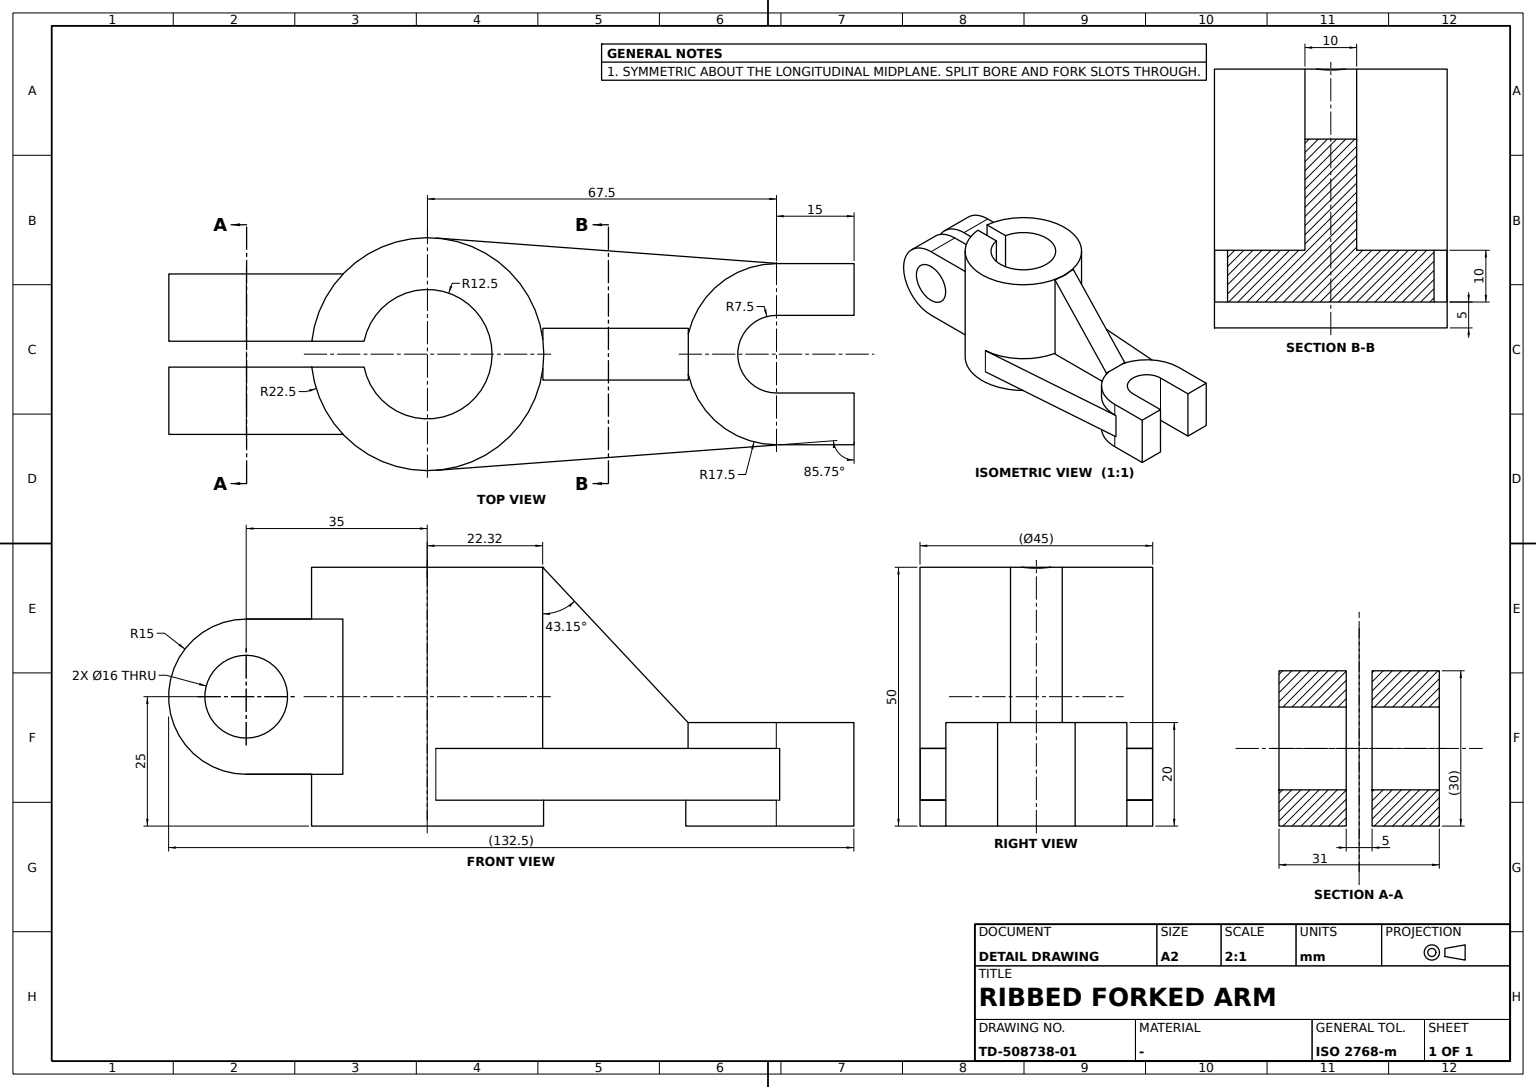
ISO-10303-21;
HEADER;
FILE_DESCRIPTION((''),'2;1');
FILE_NAME('','',(''),(''),'','','');
FILE_SCHEMA(('AUTOMOTIVE_DESIGN'));
ENDSEC;
DATA;
#1=APPLICATION_CONTEXT('');
#2=PRODUCT_CONTEXT('',#1,'mechanical');
#3=PRODUCT('','','',(#2));
#4=PRODUCT_DEFINITION_FORMATION('','',#3);
#5=PRODUCT_DEFINITION_CONTEXT('',#1,'design');
#6=PRODUCT_DEFINITION('','',#4,#5);
#7=PRODUCT_DEFINITION_SHAPE('','',#6);
#8=(LENGTH_UNIT()NAMED_UNIT(*)SI_UNIT(.MILLI.,.METRE.));
#9=(NAMED_UNIT(*)PLANE_ANGLE_UNIT()SI_UNIT($,.RADIAN.));
#10=(NAMED_UNIT(*)SI_UNIT($,.STERADIAN.)SOLID_ANGLE_UNIT());
#11=UNCERTAINTY_MEASURE_WITH_UNIT(LENGTH_MEASURE(0.005),#8,'distance_accuracy_value','');
#12=(GEOMETRIC_REPRESENTATION_CONTEXT(3)GLOBAL_UNCERTAINTY_ASSIGNED_CONTEXT((#11))GLOBAL_UNIT_ASSIGNED_CONTEXT((#8,#9,#10))REPRESENTATION_CONTEXT('',''));
#13=CARTESIAN_POINT('',(7.5,-17.5,0.));
#14=VERTEX_POINT('',#13);
#15=CARTESIAN_POINT('',(7.5,-7.5,0.));
#16=VERTEX_POINT('',#15);
#17=CARTESIAN_POINT('',(7.5,0.,0.));
#18=DIRECTION('',(0.,1.,0.));
#19=VECTOR('',#18,1000.);
#20=LINE('',#17,#19);
#21=EDGE_CURVE('',#14,#16,#20,.T.);
#22=ORIENTED_EDGE('',*,*,#21,.T.);
#23=CARTESIAN_POINT('',(7.5,-7.5,20.));
#24=VERTEX_POINT('',#23);
#25=DIRECTION('',(0.,0.,-1.));
#26=VECTOR('',#25,1000.);
#27=LINE('',#15,#26);
#28=EDGE_CURVE('',#24,#16,#27,.T.);
#29=ORIENTED_EDGE('',*,*,#28,.F.);
#30=CARTESIAN_POINT('',(7.5,-17.5,20.));
#31=VERTEX_POINT('',#30);
#32=CARTESIAN_POINT('',(7.5,0.,20.));
#33=LINE('',#32,#19);
#34=EDGE_CURVE('',#31,#24,#33,.T.);
#35=ORIENTED_EDGE('',*,*,#34,.F.);
#36=DIRECTION('',(0.,0.,1.));
#37=VECTOR('',#36,1000.);
#38=LINE('',#13,#37);
#39=EDGE_CURVE('',#14,#31,#38,.T.);
#40=ORIENTED_EDGE('',*,*,#39,.F.);
#41=EDGE_LOOP('',(#22,#29,#35,#40));
#42=FACE_BOUND('',#41,.T.);
#43=DIRECTION('',(1.,0.,0.));
#44=AXIS2_PLACEMENT_3D('',#13,#43,#18);
#45=PLANE('',#44);
#46=ADVANCED_FACE('',(#42),#45,.T.);
#47=CARTESIAN_POINT('',(-110.,2.5,33.));
#48=VERTEX_POINT('',#47);
#49=CARTESIAN_POINT('',(-110.,2.5,25.));
#50=AXIS2_PLACEMENT_3D('',#49,#18,#36);
#51=CIRCLE('',#50,8.);
#52=EDGE_CURVE('',#48,#48,#51,.T.);
#53=ORIENTED_EDGE('',*,*,#52,.F.);
#54=EDGE_LOOP('',(#53));
#55=FACE_BOUND('',#54,.T.);
#56=CARTESIAN_POINT('',(-110.,15.5,33.));
#57=VERTEX_POINT('',#56);
#58=CARTESIAN_POINT('',(-110.,15.5,25.));
#59=AXIS2_PLACEMENT_3D('',#58,#18,#36);
#60=CIRCLE('',#59,8.);
#61=EDGE_CURVE('',#57,#57,#60,.T.);
#62=ORIENTED_EDGE('',*,*,#61,.T.);
#63=EDGE_LOOP('',(#62));
#64=FACE_BOUND('',#63,.T.);
#65=CARTESIAN_POINT('',(-110.,0.,25.));
#66=DIRECTION('',(-1.,0.,0.));
#67=AXIS2_PLACEMENT_3D('',#65,#18,#66);
#68=CYLINDRICAL_SURFACE('',#67,8.);
#69=ADVANCED_FACE('',(#55,#64),#68,.F.);
#70=CARTESIAN_POINT('',(-52.67588,-2.80779,50.));
#71=VERTEX_POINT('',#70);
#72=CARTESIAN_POINT('',(-52.67588,2.80779,50.));
#73=VERTEX_POINT('',#72);
#74=CARTESIAN_POINT('',(-75.,0.,73.818335));
#75=DIRECTION('',(0.729622329,0.,0.683850318));
#76=DIRECTION('',(0.683850318,0.,-0.729622329));
#77=AXIS2_PLACEMENT_3D('',#74,#75,#76);
#78=ELLIPSE('',#77,32.901937,22.5);
#79=EDGE_CURVE('',#71,#73,#78,.T.);
#80=ORIENTED_EDGE('',*,*,#79,.T.);
#81=CARTESIAN_POINT('',(-75.,0.,50.));
#82=AXIS2_PLACEMENT_3D('',#81,#25,#66);
#83=CIRCLE('',#82,22.5);
#84=EDGE_CURVE('',#73,#71,#83,.T.);
#85=ORIENTED_EDGE('',*,*,#84,.T.);
#86=EDGE_LOOP('',(#80,#85));
#87=FACE_BOUND('',#86,.T.);
#88=CARTESIAN_POINT('',(-75.,0.,25.));
#89=AXIS2_PLACEMENT_3D('',#88,#25,#43);
#90=CYLINDRICAL_SURFACE('',#89,22.5);
#91=ADVANCED_FACE('',(#87),#90,.T.);
#92=CARTESIAN_POINT('',(-6.850961,-17.5,5.));
#93=VERTEX_POINT('',#92);
#94=CARTESIAN_POINT('',(-6.850961,-17.5,15.));
#95=VERTEX_POINT('',#94);
#96=CARTESIAN_POINT('',(-6.85096,-17.5,5.));
#97=LINE('',#96,#37);
#98=EDGE_CURVE('',#93,#95,#97,.T.);
#99=ORIENTED_EDGE('',*,*,#98,.T.);
#100=CARTESIAN_POINT('',(-7.498125,-17.523965,15.));
#101=VERTEX_POINT('',#100);
#102=CARTESIAN_POINT('',(-7.498125,-17.5,15.));
#103=CARTESIAN_POINT('',(-7.282404,-17.5,15.));
#104=CARTESIAN_POINT('',(-7.066682,-17.5,15.));
#105=B_SPLINE_CURVE_WITH_KNOTS('',3,(#102,#103,#104,#94),.UNSPECIFIED.,.F.,.F.,(4,4),(-0.322644964,0.324519594),.UNSPECIFIED.);
#106=EDGE_CURVE('',#95,#101,#105,.F.);
#107=ORIENTED_EDGE('',*,*,#106,.T.);
#108=CARTESIAN_POINT('',(-73.333333,-22.438187,15.));
#109=VERTEX_POINT('',#108);
#110=CARTESIAN_POINT('',(1.255144,-16.897894,15.));
#111=DIRECTION('',(0.997252742,0.074074074,0.));
#112=VECTOR('',#111,1000.);
#113=LINE('',#110,#112);
#114=EDGE_CURVE('',#109,#101,#113,.T.);
#115=ORIENTED_EDGE('',*,*,#114,.F.);
#116=CARTESIAN_POINT('',(-73.333333,-22.438187,5.));
#117=VERTEX_POINT('',#116);
#118=CARTESIAN_POINT('',(-73.333333,-22.438187,25.));
#119=LINE('',#118,#26);
#120=EDGE_CURVE('',#117,#109,#119,.F.);
#121=ORIENTED_EDGE('',*,*,#120,.F.);
#122=CARTESIAN_POINT('',(-7.498136,-17.523966,5.));
#123=VERTEX_POINT('',#122);
#124=CARTESIAN_POINT('',(1.255144,-16.897894,5.));
#125=LINE('',#124,#112);
#126=EDGE_CURVE('',#117,#123,#125,.T.);
#127=ORIENTED_EDGE('',*,*,#126,.T.);
#128=CARTESIAN_POINT('',(-7.066686,-17.5,5.));
#129=CARTESIAN_POINT('',(-7.282411,-17.5,5.));
#130=CARTESIAN_POINT('',(-7.498136,-17.5,5.));
#131=B_SPLINE_CURVE_WITH_KNOTS('',3,(#92,#128,#129,#130),.UNSPECIFIED.,.F.,.F.,(4,4),(-0.324519594,0.322656198),.UNSPECIFIED.);
#132=EDGE_CURVE('',#123,#93,#131,.F.);
#133=ORIENTED_EDGE('',*,*,#132,.T.);
#134=EDGE_LOOP('',(#99,#107,#115,#121,#127,#133));
#135=FACE_BOUND('',#134,.T.);
#136=DIRECTION('',(0.074074074,-0.997252742,0.));
#137=AXIS2_PLACEMENT_3D('',#116,#136,#111);
#138=PLANE('',#137);
#139=ADVANCED_FACE('',(#135),#138,.T.);
#140=CARTESIAN_POINT('',(-24.557896,-3.908733,20.));
#141=VERTEX_POINT('',#140);
#142=CARTESIAN_POINT('',(-24.557896,-3.908733,15.));
#143=VERTEX_POINT('',#142);
#144=LINE('',#142,#37);
#145=EDGE_CURVE('',#141,#143,#144,.F.);
#146=ORIENTED_EDGE('',*,*,#145,.T.);
#147=CARTESIAN_POINT('',(-7.5,0.,15.));
#148=AXIS2_PLACEMENT_3D('',#147,#36,#43);
#149=CIRCLE('',#148,17.5);
#150=EDGE_CURVE('',#143,#101,#149,.T.);
#151=ORIENTED_EDGE('',*,*,#150,.T.);
#152=CARTESIAN_POINT('',(-7.5,-17.5,20.));
#153=VERTEX_POINT('',#152);
#154=CARTESIAN_POINT('',(-7.5,-17.5,10.));
#155=LINE('',#154,#37);
#156=EDGE_CURVE('',#153,#101,#155,.F.);
#157=ORIENTED_EDGE('',*,*,#156,.F.);
#158=CARTESIAN_POINT('',(-7.5,0.,20.));
#159=AXIS2_PLACEMENT_3D('',#158,#36,#43);
#160=CIRCLE('',#159,17.5);
#161=EDGE_CURVE('',#141,#153,#160,.T.);
#162=ORIENTED_EDGE('',*,*,#161,.F.);
#163=EDGE_LOOP('',(#146,#151,#157,#162));
#164=FACE_BOUND('',#163,.T.);
#165=CARTESIAN_POINT('',(-7.5,0.,10.));
#166=AXIS2_PLACEMENT_3D('',#165,#36,#43);
#167=CYLINDRICAL_SURFACE('',#166,17.5);
#168=ADVANCED_FACE('',(#164),#167,.T.);
#169=CARTESIAN_POINT('',(-24.557896,5.,15.));
#170=VERTEX_POINT('',#169);
#171=CARTESIAN_POINT('',(-52.67588,5.,15.));
#172=VERTEX_POINT('',#171);
#173=CARTESIAN_POINT('',(0.,5.,15.));
#174=VECTOR('',#66,1000.);
#175=LINE('',#173,#174);
#176=EDGE_CURVE('',#170,#172,#175,.T.);
#177=ORIENTED_EDGE('',*,*,#176,.T.);
#178=CARTESIAN_POINT('',(-52.67588,5.,50.));
#179=VERTEX_POINT('',#178);
#180=CARTESIAN_POINT('',(-52.67588,5.,0.));
#181=LINE('',#180,#37);
#182=EDGE_CURVE('',#172,#179,#181,.T.);
#183=ORIENTED_EDGE('',*,*,#182,.T.);
#184=CARTESIAN_POINT('',(-24.557896,5.,20.));
#185=VERTEX_POINT('',#184);
#186=CARTESIAN_POINT('',(-3.094316,5.,-2.900197));
#187=VECTOR('',#76,1000.);
#188=LINE('',#186,#187);
#189=EDGE_CURVE('',#179,#185,#188,.T.);
#190=ORIENTED_EDGE('',*,*,#189,.T.);
#191=CARTESIAN_POINT('',(-24.557896,5.,0.));
#192=LINE('',#191,#26);
#193=EDGE_CURVE('',#185,#170,#192,.T.);
#194=ORIENTED_EDGE('',*,*,#193,.T.);
#195=EDGE_LOOP('',(#177,#183,#190,#194));
#196=FACE_BOUND('',#195,.T.);
#197=CARTESIAN_POINT('',(0.,5.,0.));
#198=AXIS2_PLACEMENT_3D('',#197,#18,#66);
#199=PLANE('',#198);
#200=ADVANCED_FACE('',(#196),#199,.T.);
#201=CARTESIAN_POINT('',(-7.5,-17.5,0.));
#202=VERTEX_POINT('',#201);
#203=EDGE_CURVE('',#123,#202,#155,.F.);
#204=ORIENTED_EDGE('',*,*,#203,.F.);
#205=CARTESIAN_POINT('',(-7.498107,17.523964,5.));
#206=VERTEX_POINT('',#205);
#207=CARTESIAN_POINT('',(-7.5,0.,5.));
#208=AXIS2_PLACEMENT_3D('',#207,#36,#43);
#209=CIRCLE('',#208,17.5);
#210=EDGE_CURVE('',#206,#123,#209,.T.);
#211=ORIENTED_EDGE('',*,*,#210,.F.);
#212=CARTESIAN_POINT('',(-7.5,17.5,0.));
#213=VERTEX_POINT('',#212);
#214=CARTESIAN_POINT('',(-7.5,17.5,10.));
#215=LINE('',#214,#37);
#216=EDGE_CURVE('',#206,#213,#215,.F.);
#217=ORIENTED_EDGE('',*,*,#216,.T.);
#218=CARTESIAN_POINT('',(-7.5,0.,0.));
#219=AXIS2_PLACEMENT_3D('',#218,#36,#43);
#220=CIRCLE('',#219,17.5);
#221=EDGE_CURVE('',#213,#202,#220,.T.);
#222=ORIENTED_EDGE('',*,*,#221,.T.);
#223=EDGE_LOOP('',(#204,#211,#217,#222));
#224=FACE_BOUND('',#223,.T.);
#225=ADVANCED_FACE('',(#224),#167,.T.);
#226=CARTESIAN_POINT('',(-52.67588,2.80779,15.));
#227=VERTEX_POINT('',#226);
#228=CARTESIAN_POINT('',(-52.67588,0.,15.));
#229=LINE('',#228,#19);
#230=EDGE_CURVE('',#227,#172,#229,.T.);
#231=ORIENTED_EDGE('',*,*,#230,.F.);
#232=LINE('',#72,#26);
#233=EDGE_CURVE('',#73,#227,#232,.T.);
#234=ORIENTED_EDGE('',*,*,#233,.F.);
#235=CARTESIAN_POINT('',(-52.67588,0.,50.));
#236=LINE('',#235,#19);
#237=EDGE_CURVE('',#73,#179,#236,.T.);
#238=ORIENTED_EDGE('',*,*,#237,.T.);
#239=ORIENTED_EDGE('',*,*,#182,.F.);
#240=EDGE_LOOP('',(#231,#234,#238,#239));
#241=FACE_BOUND('',#240,.T.);
#242=AXIS2_PLACEMENT_3D('',#228,#66,#36);
#243=PLANE('',#242);
#244=ADVANCED_FACE('',(#241),#243,.T.);
#245=CARTESIAN_POINT('',(-24.557896,-5.,15.));
#246=VERTEX_POINT('',#245);
#247=CARTESIAN_POINT('',(-24.557896,0.,15.));
#248=LINE('',#247,#19);
#249=EDGE_CURVE('',#246,#143,#248,.T.);
#250=ORIENTED_EDGE('',*,*,#249,.T.);
#251=ORIENTED_EDGE('',*,*,#145,.F.);
#252=CARTESIAN_POINT('',(-24.557896,-5.,20.));
#253=VERTEX_POINT('',#252);
#254=CARTESIAN_POINT('',(-24.557896,0.,20.));
#255=LINE('',#254,#19);
#256=EDGE_CURVE('',#253,#141,#255,.T.);
#257=ORIENTED_EDGE('',*,*,#256,.F.);
#258=CARTESIAN_POINT('',(-24.557896,-5.,0.));
#259=LINE('',#258,#26);
#260=EDGE_CURVE('',#253,#246,#259,.T.);
#261=ORIENTED_EDGE('',*,*,#260,.T.);
#262=EDGE_LOOP('',(#250,#251,#257,#261));
#263=FACE_BOUND('',#262,.T.);
#264=AXIS2_PLACEMENT_3D('',#254,#43,#25);
#265=PLANE('',#264);
#266=ADVANCED_FACE('',(#263),#265,.T.);
#267=CARTESIAN_POINT('',(-97.36068,2.5,0.));
#268=VERTEX_POINT('',#267);
#269=CARTESIAN_POINT('',(-97.36068,-2.5,0.));
#270=VERTEX_POINT('',#269);
#271=CARTESIAN_POINT('',(-75.,0.,0.));
#272=AXIS2_PLACEMENT_3D('',#271,#36,#43);
#273=CIRCLE('',#272,22.5);
#274=EDGE_CURVE('',#268,#270,#273,.F.);
#275=ORIENTED_EDGE('',*,*,#274,.T.);
#276=CARTESIAN_POINT('',(-87.247449,-2.5,0.));
#277=VERTEX_POINT('',#276);
#278=CARTESIAN_POINT('',(-85.978546,-2.5,0.));
#279=LINE('',#278,#174);
#280=EDGE_CURVE('',#277,#270,#279,.T.);
#281=ORIENTED_EDGE('',*,*,#280,.F.);
#282=CARTESIAN_POINT('',(-87.247449,2.5,0.));
#283=VERTEX_POINT('',#282);
#284=CIRCLE('',#272,12.5);
#285=EDGE_CURVE('',#283,#277,#284,.F.);
#286=ORIENTED_EDGE('',*,*,#285,.F.);
#287=CARTESIAN_POINT('',(0.,2.5,0.));
#288=LINE('',#287,#174);
#289=EDGE_CURVE('',#283,#268,#288,.T.);
#290=ORIENTED_EDGE('',*,*,#289,.T.);
#291=EDGE_LOOP('',(#275,#281,#286,#290));
#292=FACE_BOUND('',#291,.T.);
#293=CARTESIAN_POINT('',(0.,0.,0.));
#294=AXIS2_PLACEMENT_3D('',#293,#36,#43);
#295=PLANE('',#294);
#296=ADVANCED_FACE('',(#292),#295,.F.);
#297=CARTESIAN_POINT('',(-87.247449,-2.5,50.));
#298=VERTEX_POINT('',#297);
#299=CARTESIAN_POINT('',(-97.36068,-2.5,50.));
#300=VERTEX_POINT('',#299);
#301=CARTESIAN_POINT('',(0.,-2.5,50.));
#302=LINE('',#301,#174);
#303=EDGE_CURVE('',#298,#300,#302,.T.);
#304=ORIENTED_EDGE('',*,*,#303,.T.);
#305=EDGE_CURVE('',#71,#300,#83,.T.);
#306=ORIENTED_EDGE('',*,*,#305,.F.);
#307=ORIENTED_EDGE('',*,*,#84,.F.);
#308=CARTESIAN_POINT('',(-97.36068,2.5,50.));
#309=VERTEX_POINT('',#308);
#310=EDGE_CURVE('',#309,#73,#83,.T.);
#311=ORIENTED_EDGE('',*,*,#310,.F.);
#312=CARTESIAN_POINT('',(-87.247449,2.5,50.));
#313=VERTEX_POINT('',#312);
#314=CARTESIAN_POINT('',(0.,2.5,50.));
#315=VECTOR('',#43,1000.);
#316=LINE('',#314,#315);
#317=EDGE_CURVE('',#309,#313,#316,.T.);
#318=ORIENTED_EDGE('',*,*,#317,.T.);
#319=CIRCLE('',#82,12.5);
#320=EDGE_CURVE('',#313,#298,#319,.T.);
#321=ORIENTED_EDGE('',*,*,#320,.T.);
#322=EDGE_LOOP('',(#304,#306,#307,#311,#318,#321));
#323=FACE_BOUND('',#322,.T.);
#324=CARTESIAN_POINT('',(0.,0.,50.));
#325=AXIS2_PLACEMENT_3D('',#324,#25,#43);
#326=PLANE('',#325);
#327=ADVANCED_FACE('',(#323),#326,.F.);
#328=CARTESIAN_POINT('',(-52.67588,-5.,15.));
#329=VERTEX_POINT('',#328);
#330=CARTESIAN_POINT('',(0.,-5.,15.));
#331=LINE('',#330,#174);
#332=EDGE_CURVE('',#246,#329,#331,.T.);
#333=ORIENTED_EDGE('',*,*,#332,.T.);
#334=CARTESIAN_POINT('',(-52.67588,-2.80779,15.));
#335=VERTEX_POINT('',#334);
#336=EDGE_CURVE('',#329,#335,#229,.T.);
#337=ORIENTED_EDGE('',*,*,#336,.T.);
#338=CARTESIAN_POINT('',(-75.,0.,15.));
#339=AXIS2_PLACEMENT_3D('',#338,#36,#43);
#340=CIRCLE('',#339,22.5);
#341=EDGE_CURVE('',#109,#335,#340,.T.);
#342=ORIENTED_EDGE('',*,*,#341,.F.);
#343=ORIENTED_EDGE('',*,*,#114,.T.);
#344=ORIENTED_EDGE('',*,*,#150,.F.);
#345=ORIENTED_EDGE('',*,*,#249,.F.);
#346=EDGE_LOOP('',(#333,#337,#342,#343,#344,#345));
#347=FACE_BOUND('',#346,.T.);
#348=CARTESIAN_POINT('',(0.,0.,15.));
#349=AXIS2_PLACEMENT_3D('',#348,#36,#43);
#350=PLANE('',#349);
#351=ADVANCED_FACE('',(#347),#350,.T.);
#352=CARTESIAN_POINT('',(-52.67588,-5.,50.));
#353=VERTEX_POINT('',#352);
#354=EDGE_CURVE('',#353,#71,#236,.T.);
#355=ORIENTED_EDGE('',*,*,#354,.F.);
#356=CARTESIAN_POINT('',(-3.094316,-5.,-2.900197));
#357=LINE('',#356,#187);
#358=EDGE_CURVE('',#353,#253,#357,.T.);
#359=ORIENTED_EDGE('',*,*,#358,.T.);
#360=ORIENTED_EDGE('',*,*,#256,.T.);
#361=CARTESIAN_POINT('',(-24.557896,3.908733,20.));
#362=VERTEX_POINT('',#361);
#363=DIRECTION('',(0.,-1.,0.));
#364=VECTOR('',#363,1000.);
#365=LINE('',#254,#364);
#366=EDGE_CURVE('',#362,#141,#365,.T.);
#367=ORIENTED_EDGE('',*,*,#366,.F.);
#368=EDGE_CURVE('',#362,#185,#255,.T.);
#369=ORIENTED_EDGE('',*,*,#368,.T.);
#370=ORIENTED_EDGE('',*,*,#189,.F.);
#371=ORIENTED_EDGE('',*,*,#237,.F.);
#372=ORIENTED_EDGE('',*,*,#79,.F.);
#373=EDGE_LOOP('',(#355,#359,#360,#367,#369,#370,#371,#372));
#374=FACE_BOUND('',#373,.T.);
#375=AXIS2_PLACEMENT_3D('',#235,#75,#76);
#376=PLANE('',#375);
#377=ADVANCED_FACE('',(#374),#376,.T.);
#378=ORIENTED_EDGE('',*,*,#28,.T.);
#379=CARTESIAN_POINT('',(-7.5,-7.5,0.));
#380=VERTEX_POINT('',#379);
#381=LINE('',#15,#174);
#382=EDGE_CURVE('',#16,#380,#381,.T.);
#383=ORIENTED_EDGE('',*,*,#382,.T.);
#384=CARTESIAN_POINT('',(-7.5,-7.5,20.));
#385=VERTEX_POINT('',#384);
#386=CARTESIAN_POINT('',(-7.5,-7.5,10.));
#387=LINE('',#386,#37);
#388=EDGE_CURVE('',#385,#380,#387,.F.);
#389=ORIENTED_EDGE('',*,*,#388,.F.);
#390=LINE('',#23,#174);
#391=EDGE_CURVE('',#24,#385,#390,.T.);
#392=ORIENTED_EDGE('',*,*,#391,.F.);
#393=EDGE_LOOP('',(#378,#383,#389,#392));
#394=FACE_BOUND('',#393,.T.);
#395=AXIS2_PLACEMENT_3D('',#23,#363,#66);
#396=PLANE('',#395);
#397=ADVANCED_FACE('',(#394),#396,.F.);
#398=CARTESIAN_POINT('',(-110.,-2.5,17.));
#399=VERTEX_POINT('',#398);
#400=CARTESIAN_POINT('',(-110.,-2.5,25.));
#401=AXIS2_PLACEMENT_3D('',#400,#363,#25);
#402=CIRCLE('',#401,8.);
#403=EDGE_CURVE('',#399,#399,#402,.T.);
#404=ORIENTED_EDGE('',*,*,#403,.T.);
#405=EDGE_LOOP('',(#404));
#406=FACE_BOUND('',#405,.T.);
#407=CARTESIAN_POINT('',(-97.36068,-2.5,40.));
#408=VERTEX_POINT('',#407);
#409=LINE('',#299,#26);
#410=EDGE_CURVE('',#300,#408,#409,.T.);
#411=ORIENTED_EDGE('',*,*,#410,.F.);
#412=ORIENTED_EDGE('',*,*,#303,.F.);
#413=CARTESIAN_POINT('',(-87.247449,-2.5,10.));
#414=LINE('',#413,#37);
#415=EDGE_CURVE('',#277,#298,#414,.T.);
#416=ORIENTED_EDGE('',*,*,#415,.F.);
#417=ORIENTED_EDGE('',*,*,#280,.T.);
#418=CARTESIAN_POINT('',(-97.36068,-2.5,10.));
#419=VERTEX_POINT('',#418);
#420=LINE('',#418,#26);
#421=EDGE_CURVE('',#419,#270,#420,.T.);
#422=ORIENTED_EDGE('',*,*,#421,.F.);
#423=CARTESIAN_POINT('',(-110.,-2.5,10.));
#424=VERTEX_POINT('',#423);
#425=LINE('',#423,#315);
#426=EDGE_CURVE('',#424,#419,#425,.T.);
#427=ORIENTED_EDGE('',*,*,#426,.F.);
#428=CARTESIAN_POINT('',(-110.,-2.5,40.));
#429=VERTEX_POINT('',#428);
#430=CIRCLE('',#401,15.);
#431=EDGE_CURVE('',#429,#424,#430,.T.);
#432=ORIENTED_EDGE('',*,*,#431,.F.);
#433=CARTESIAN_POINT('',(-75.,-2.5,40.));
#434=LINE('',#433,#174);
#435=EDGE_CURVE('',#408,#429,#434,.T.);
#436=ORIENTED_EDGE('',*,*,#435,.F.);
#437=EDGE_LOOP('',(#411,#412,#416,#417,#422,#427,#432,#436));
#438=FACE_BOUND('',#437,.T.);
#439=CARTESIAN_POINT('',(-85.978546,-2.5,50.));
#440=AXIS2_PLACEMENT_3D('',#439,#363,#66);
#441=PLANE('',#440);
#442=ADVANCED_FACE('',(#406,#438),#441,.F.);
#443=ORIENTED_EDGE('',*,*,#221,.F.);
#444=CARTESIAN_POINT('',(7.5,17.5,0.));
#445=VERTEX_POINT('',#444);
#446=CARTESIAN_POINT('',(0.,17.5,0.));
#447=LINE('',#446,#315);
#448=EDGE_CURVE('',#213,#445,#447,.T.);
#449=ORIENTED_EDGE('',*,*,#448,.T.);
#450=CARTESIAN_POINT('',(7.5,7.5,0.));
#451=VERTEX_POINT('',#450);
#452=EDGE_CURVE('',#451,#445,#20,.T.);
#453=ORIENTED_EDGE('',*,*,#452,.F.);
#454=CARTESIAN_POINT('',(-7.5,7.5,0.));
#455=VERTEX_POINT('',#454);
#456=LINE('',#454,#315);
#457=EDGE_CURVE('',#455,#451,#456,.T.);
#458=ORIENTED_EDGE('',*,*,#457,.F.);
#459=CIRCLE('',#219,7.5);
#460=EDGE_CURVE('',#455,#380,#459,.T.);
#461=ORIENTED_EDGE('',*,*,#460,.T.);
#462=ORIENTED_EDGE('',*,*,#382,.F.);
#463=ORIENTED_EDGE('',*,*,#21,.F.);
#464=CARTESIAN_POINT('',(0.,-17.5,0.));
#465=LINE('',#464,#174);
#466=EDGE_CURVE('',#14,#202,#465,.T.);
#467=ORIENTED_EDGE('',*,*,#466,.T.);
#468=EDGE_LOOP('',(#443,#449,#453,#458,#461,#462,#463,#467));
#469=FACE_BOUND('',#468,.T.);
#470=ADVANCED_FACE('',(#469),#295,.F.);
#471=CARTESIAN_POINT('',(-6.850961,17.5,5.));
#472=VERTEX_POINT('',#471);
#473=CARTESIAN_POINT('',(-7.498107,17.5,5.));
#474=CARTESIAN_POINT('',(-7.282391,17.5,5.));
#475=CARTESIAN_POINT('',(-7.066676,17.5,5.));
#476=B_SPLINE_CURVE_WITH_KNOTS('',3,(#473,#474,#475,#471),.UNSPECIFIED.,.F.,.F.,(4,4),(-0.322626491,0.324519594),.UNSPECIFIED.);
#477=EDGE_CURVE('',#472,#206,#476,.F.);
#478=ORIENTED_EDGE('',*,*,#477,.T.);
#479=CARTESIAN_POINT('',(-73.333333,22.438187,5.));
#480=VERTEX_POINT('',#479);
#481=CARTESIAN_POINT('',(1.255144,16.897894,5.));
#482=DIRECTION('',(0.997252742,-0.074074074,0.));
#483=VECTOR('',#482,1000.);
#484=LINE('',#481,#483);
#485=EDGE_CURVE('',#480,#206,#484,.T.);
#486=ORIENTED_EDGE('',*,*,#485,.F.);
#487=CARTESIAN_POINT('',(-73.333333,22.438187,15.));
#488=VERTEX_POINT('',#487);
#489=CARTESIAN_POINT('',(-73.333333,22.438187,25.));
#490=LINE('',#489,#26);
#491=EDGE_CURVE('',#480,#488,#490,.F.);
#492=ORIENTED_EDGE('',*,*,#491,.T.);
#493=CARTESIAN_POINT('',(-7.498136,17.523966,15.));
#494=VERTEX_POINT('',#493);
#495=CARTESIAN_POINT('',(1.255144,16.897894,15.));
#496=LINE('',#495,#483);
#497=EDGE_CURVE('',#488,#494,#496,.T.);
#498=ORIENTED_EDGE('',*,*,#497,.T.);
#499=CARTESIAN_POINT('',(-6.850961,17.5,15.));
#500=VERTEX_POINT('',#499);
#501=CARTESIAN_POINT('',(-7.066686,17.5,15.));
#502=CARTESIAN_POINT('',(-7.282411,17.5,15.));
#503=CARTESIAN_POINT('',(-7.498136,17.5,15.));
#504=B_SPLINE_CURVE_WITH_KNOTS('',3,(#499,#501,#502,#503),.UNSPECIFIED.,.F.,.F.,(4,4),(-0.324519594,0.322656194),.UNSPECIFIED.);
#505=EDGE_CURVE('',#494,#500,#504,.F.);
#506=ORIENTED_EDGE('',*,*,#505,.T.);
#507=CARTESIAN_POINT('',(-6.85096,17.5,5.));
#508=LINE('',#507,#37);
#509=EDGE_CURVE('',#500,#472,#508,.F.);
#510=ORIENTED_EDGE('',*,*,#509,.T.);
#511=EDGE_LOOP('',(#478,#486,#492,#498,#506,#510));
#512=FACE_BOUND('',#511,.T.);
#513=DIRECTION('',(-0.074074074,-0.997252742,0.));
#514=AXIS2_PLACEMENT_3D('',#479,#513,#482);
#515=PLANE('',#514);
#516=ADVANCED_FACE('',(#512),#515,.F.);
#517=CARTESIAN_POINT('',(-91.309506,-15.5,10.));
#518=VERTEX_POINT('',#517);
#519=CARTESIAN_POINT('',(-75.,0.,10.));
#520=AXIS2_PLACEMENT_3D('',#519,#36,#43);
#521=CIRCLE('',#520,22.5);
#522=EDGE_CURVE('',#419,#518,#521,.T.);
#523=ORIENTED_EDGE('',*,*,#522,.T.);
#524=CARTESIAN_POINT('',(-110.,-15.5,10.));
#525=VERTEX_POINT('',#524);
#526=CARTESIAN_POINT('',(0.,-15.5,10.));
#527=LINE('',#526,#315);
#528=EDGE_CURVE('',#525,#518,#527,.T.);
#529=ORIENTED_EDGE('',*,*,#528,.F.);
#530=CARTESIAN_POINT('',(-110.,0.,10.));
#531=LINE('',#530,#19);
#532=EDGE_CURVE('',#424,#525,#531,.F.);
#533=ORIENTED_EDGE('',*,*,#532,.F.);
#534=ORIENTED_EDGE('',*,*,#426,.T.);
#535=EDGE_LOOP('',(#523,#529,#533,#534));
#536=FACE_BOUND('',#535,.T.);
#537=AXIS2_PLACEMENT_3D('',#530,#36,#43);
#538=PLANE('',#537);
#539=ADVANCED_FACE('',(#536),#538,.F.);
#540=CARTESIAN_POINT('',(-110.,-15.5,33.));
#541=VERTEX_POINT('',#540);
#542=CARTESIAN_POINT('',(-110.,-15.5,25.));
#543=AXIS2_PLACEMENT_3D('',#542,#18,#36);
#544=CIRCLE('',#543,8.);
#545=EDGE_CURVE('',#541,#541,#544,.T.);
#546=ORIENTED_EDGE('',*,*,#545,.T.);
#547=EDGE_LOOP('',(#546));
#548=FACE_BOUND('',#547,.T.);
#549=CARTESIAN_POINT('',(-91.309506,-15.5,40.));
#550=VERTEX_POINT('',#549);
#551=LINE('',#517,#26);
#552=EDGE_CURVE('',#518,#550,#551,.F.);
#553=ORIENTED_EDGE('',*,*,#552,.T.);
#554=CARTESIAN_POINT('',(-110.,-15.5,40.));
#555=VERTEX_POINT('',#554);
#556=CARTESIAN_POINT('',(0.,-15.5,40.));
#557=LINE('',#556,#174);
#558=EDGE_CURVE('',#550,#555,#557,.T.);
#559=ORIENTED_EDGE('',*,*,#558,.T.);
#560=CIRCLE('',#543,15.);
#561=EDGE_CURVE('',#525,#555,#560,.T.);
#562=ORIENTED_EDGE('',*,*,#561,.F.);
#563=ORIENTED_EDGE('',*,*,#528,.T.);
#564=EDGE_LOOP('',(#553,#559,#562,#563));
#565=FACE_BOUND('',#564,.T.);
#566=CARTESIAN_POINT('',(0.,-15.5,0.));
#567=AXIS2_PLACEMENT_3D('',#566,#18,#66);
#568=PLANE('',#567);
#569=ADVANCED_FACE('',(#548,#565),#568,.F.);
#570=CARTESIAN_POINT('',(-110.,2.5,10.));
#571=VERTEX_POINT('',#570);
#572=CARTESIAN_POINT('',(-110.,2.5,40.));
#573=VERTEX_POINT('',#572);
#574=CIRCLE('',#50,15.);
#575=EDGE_CURVE('',#571,#573,#574,.T.);
#576=ORIENTED_EDGE('',*,*,#575,.F.);
#577=CARTESIAN_POINT('',(-97.36068,2.5,10.));
#578=VERTEX_POINT('',#577);
#579=CARTESIAN_POINT('',(-129.238556,2.5,10.));
#580=LINE('',#579,#315);
#581=EDGE_CURVE('',#571,#578,#580,.T.);
#582=ORIENTED_EDGE('',*,*,#581,.T.);
#583=LINE('',#577,#26);
#584=EDGE_CURVE('',#578,#268,#583,.T.);
#585=ORIENTED_EDGE('',*,*,#584,.T.);
#586=ORIENTED_EDGE('',*,*,#289,.F.);
#587=LINE('',#312,#37);
#588=EDGE_CURVE('',#313,#283,#587,.F.);
#589=ORIENTED_EDGE('',*,*,#588,.F.);
#590=ORIENTED_EDGE('',*,*,#317,.F.);
#591=CARTESIAN_POINT('',(-97.36068,2.5,40.));
#592=VERTEX_POINT('',#591);
#593=LINE('',#308,#26);
#594=EDGE_CURVE('',#309,#592,#593,.T.);
#595=ORIENTED_EDGE('',*,*,#594,.T.);
#596=CARTESIAN_POINT('',(-129.238556,2.5,40.));
#597=LINE('',#596,#174);
#598=EDGE_CURVE('',#592,#573,#597,.T.);
#599=ORIENTED_EDGE('',*,*,#598,.T.);
#600=EDGE_LOOP('',(#576,#582,#585,#586,#589,#590,#595,#599));
#601=FACE_BOUND('',#600,.T.);
#602=ORIENTED_EDGE('',*,*,#52,.T.);
#603=EDGE_LOOP('',(#602));
#604=FACE_BOUND('',#603,.T.);
#605=CARTESIAN_POINT('',(-129.238556,2.5,50.));
#606=AXIS2_PLACEMENT_3D('',#605,#18,#43);
#607=PLANE('',#606);
#608=ADVANCED_FACE('',(#601,#604),#607,.F.);
#609=EDGE_CURVE('',#227,#488,#340,.T.);
#610=ORIENTED_EDGE('',*,*,#609,.F.);
#611=ORIENTED_EDGE('',*,*,#230,.T.);
#612=ORIENTED_EDGE('',*,*,#176,.F.);
#613=CARTESIAN_POINT('',(-24.557896,3.908733,15.));
#614=VERTEX_POINT('',#613);
#615=EDGE_CURVE('',#614,#170,#248,.T.);
#616=ORIENTED_EDGE('',*,*,#615,.F.);
#617=EDGE_CURVE('',#494,#614,#149,.T.);
#618=ORIENTED_EDGE('',*,*,#617,.F.);
#619=ORIENTED_EDGE('',*,*,#497,.F.);
#620=EDGE_LOOP('',(#610,#611,#612,#616,#618,#619));
#621=FACE_BOUND('',#620,.T.);
#622=ADVANCED_FACE('',(#621),#350,.T.);
#623=ORIENTED_EDGE('',*,*,#403,.F.);
#624=EDGE_LOOP('',(#623));
#625=FACE_BOUND('',#624,.T.);
#626=ORIENTED_EDGE('',*,*,#545,.F.);
#627=EDGE_LOOP('',(#626));
#628=FACE_BOUND('',#627,.T.);
#629=ADVANCED_FACE('',(#625,#628),#68,.F.);
#630=ORIENTED_EDGE('',*,*,#61,.F.);
#631=EDGE_LOOP('',(#630));
#632=FACE_BOUND('',#631,.T.);
#633=CARTESIAN_POINT('',(-91.309506,15.5,10.));
#634=VERTEX_POINT('',#633);
#635=CARTESIAN_POINT('',(-91.309506,15.5,40.));
#636=VERTEX_POINT('',#635);
#637=LINE('',#633,#26);
#638=EDGE_CURVE('',#634,#636,#637,.F.);
#639=ORIENTED_EDGE('',*,*,#638,.F.);
#640=CARTESIAN_POINT('',(-110.,15.5,10.));
#641=VERTEX_POINT('',#640);
#642=CARTESIAN_POINT('',(0.,15.5,10.));
#643=LINE('',#642,#315);
#644=EDGE_CURVE('',#641,#634,#643,.T.);
#645=ORIENTED_EDGE('',*,*,#644,.F.);
#646=CARTESIAN_POINT('',(-110.,15.5,40.));
#647=VERTEX_POINT('',#646);
#648=CIRCLE('',#59,15.);
#649=EDGE_CURVE('',#641,#647,#648,.T.);
#650=ORIENTED_EDGE('',*,*,#649,.T.);
#651=CARTESIAN_POINT('',(0.,15.5,40.));
#652=LINE('',#651,#174);
#653=EDGE_CURVE('',#636,#647,#652,.T.);
#654=ORIENTED_EDGE('',*,*,#653,.F.);
#655=EDGE_LOOP('',(#639,#645,#650,#654));
#656=FACE_BOUND('',#655,.T.);
#657=CARTESIAN_POINT('',(0.,15.5,0.));
#658=AXIS2_PLACEMENT_3D('',#657,#18,#66);
#659=PLANE('',#658);
#660=ADVANCED_FACE('',(#632,#656),#659,.T.);
#661=ORIENTED_EDGE('',*,*,#126,.F.);
#662=CARTESIAN_POINT('',(-75.,0.,5.));
#663=AXIS2_PLACEMENT_3D('',#662,#36,#43);
#664=CIRCLE('',#663,22.5);
#665=EDGE_CURVE('',#117,#480,#664,.T.);
#666=ORIENTED_EDGE('',*,*,#665,.T.);
#667=ORIENTED_EDGE('',*,*,#485,.T.);
#668=ORIENTED_EDGE('',*,*,#210,.T.);
#669=EDGE_LOOP('',(#661,#666,#667,#668));
#670=FACE_BOUND('',#669,.T.);
#671=CARTESIAN_POINT('',(0.,0.,5.));
#672=AXIS2_PLACEMENT_3D('',#671,#36,#43);
#673=PLANE('',#672);
#674=ADVANCED_FACE('',(#670),#673,.F.);
#675=ORIENTED_EDGE('',*,*,#575,.T.);
#676=CARTESIAN_POINT('',(-110.,0.,40.));
#677=LINE('',#676,#19);
#678=EDGE_CURVE('',#647,#573,#677,.F.);
#679=ORIENTED_EDGE('',*,*,#678,.F.);
#680=ORIENTED_EDGE('',*,*,#649,.F.);
#681=EDGE_CURVE('',#641,#571,#531,.F.);
#682=ORIENTED_EDGE('',*,*,#681,.T.);
#683=EDGE_LOOP('',(#675,#679,#680,#682));
#684=FACE_BOUND('',#683,.T.);
#685=CYLINDRICAL_SURFACE('',#67,15.);
#686=ADVANCED_FACE('',(#684),#685,.T.);
#687=CARTESIAN_POINT('',(7.5,7.5,20.));
#688=VERTEX_POINT('',#687);
#689=LINE('',#687,#26);
#690=EDGE_CURVE('',#688,#451,#689,.T.);
#691=ORIENTED_EDGE('',*,*,#690,.F.);
#692=CARTESIAN_POINT('',(-7.5,7.5,20.));
#693=VERTEX_POINT('',#692);
#694=LINE('',#692,#315);
#695=EDGE_CURVE('',#693,#688,#694,.T.);
#696=ORIENTED_EDGE('',*,*,#695,.F.);
#697=CARTESIAN_POINT('',(-7.5,7.5,10.));
#698=LINE('',#697,#37);
#699=EDGE_CURVE('',#693,#455,#698,.F.);
#700=ORIENTED_EDGE('',*,*,#699,.T.);
#701=ORIENTED_EDGE('',*,*,#457,.T.);
#702=EDGE_LOOP('',(#691,#696,#700,#701));
#703=FACE_BOUND('',#702,.T.);
#704=AXIS2_PLACEMENT_3D('',#692,#18,#43);
#705=PLANE('',#704);
#706=ADVANCED_FACE('',(#703),#705,.F.);
#707=ORIENTED_EDGE('',*,*,#415,.T.);
#708=ORIENTED_EDGE('',*,*,#320,.F.);
#709=ORIENTED_EDGE('',*,*,#588,.T.);
#710=ORIENTED_EDGE('',*,*,#285,.T.);
#711=EDGE_LOOP('',(#707,#708,#709,#710));
#712=FACE_BOUND('',#711,.T.);
#713=CARTESIAN_POINT('',(-75.,0.,24.34));
#714=AXIS2_PLACEMENT_3D('',#713,#36,#43);
#715=CYLINDRICAL_SURFACE('',#714,12.5);
#716=ADVANCED_FACE('',(#712),#715,.F.);
#717=ORIENTED_EDGE('',*,*,#332,.F.);
#718=ORIENTED_EDGE('',*,*,#260,.F.);
#719=ORIENTED_EDGE('',*,*,#358,.F.);
#720=CARTESIAN_POINT('',(-52.67588,-5.,0.));
#721=LINE('',#720,#37);
#722=EDGE_CURVE('',#329,#353,#721,.T.);
#723=ORIENTED_EDGE('',*,*,#722,.F.);
#724=EDGE_LOOP('',(#717,#718,#719,#723));
#725=FACE_BOUND('',#724,.T.);
#726=CARTESIAN_POINT('',(0.,-5.,0.));
#727=AXIS2_PLACEMENT_3D('',#726,#18,#66);
#728=PLANE('',#727);
#729=ADVANCED_FACE('',(#725),#728,.F.);
#730=ORIENTED_EDGE('',*,*,#466,.F.);
#731=ORIENTED_EDGE('',*,*,#39,.T.);
#732=CARTESIAN_POINT('',(0.,-17.5,20.));
#733=LINE('',#732,#174);
#734=EDGE_CURVE('',#31,#153,#733,.T.);
#735=ORIENTED_EDGE('',*,*,#734,.T.);
#736=ORIENTED_EDGE('',*,*,#156,.T.);
#737=ORIENTED_EDGE('',*,*,#106,.F.);
#738=ORIENTED_EDGE('',*,*,#98,.F.);
#739=ORIENTED_EDGE('',*,*,#132,.F.);
#740=ORIENTED_EDGE('',*,*,#203,.T.);
#741=EDGE_LOOP('',(#730,#731,#735,#736,#737,#738,#739,#740));
#742=FACE_BOUND('',#741,.T.);
#743=AXIS2_PLACEMENT_3D('',#13,#18,#66);
#744=PLANE('',#743);
#745=ADVANCED_FACE('',(#742),#744,.F.);
#746=ORIENTED_EDGE('',*,*,#505,.F.);
#747=CARTESIAN_POINT('',(-7.5,17.5,20.));
#748=VERTEX_POINT('',#747);
#749=EDGE_CURVE('',#748,#494,#215,.F.);
#750=ORIENTED_EDGE('',*,*,#749,.F.);
#751=CARTESIAN_POINT('',(7.5,17.5,20.));
#752=VERTEX_POINT('',#751);
#753=CARTESIAN_POINT('',(0.,17.5,20.));
#754=LINE('',#753,#315);
#755=EDGE_CURVE('',#748,#752,#754,.T.);
#756=ORIENTED_EDGE('',*,*,#755,.T.);
#757=LINE('',#444,#37);
#758=EDGE_CURVE('',#445,#752,#757,.T.);
#759=ORIENTED_EDGE('',*,*,#758,.F.);
#760=ORIENTED_EDGE('',*,*,#448,.F.);
#761=ORIENTED_EDGE('',*,*,#216,.F.);
#762=ORIENTED_EDGE('',*,*,#477,.F.);
#763=ORIENTED_EDGE('',*,*,#509,.F.);
#764=EDGE_LOOP('',(#746,#750,#756,#759,#760,#761,#762,#763));
#765=FACE_BOUND('',#764,.T.);
#766=AXIS2_PLACEMENT_3D('',#212,#363,#43);
#767=PLANE('',#766);
#768=ADVANCED_FACE('',(#765),#767,.F.);
#769=ORIENTED_EDGE('',*,*,#678,.T.);
#770=ORIENTED_EDGE('',*,*,#598,.F.);
#771=CARTESIAN_POINT('',(-75.,0.,40.));
#772=AXIS2_PLACEMENT_3D('',#771,#25,#66);
#773=CIRCLE('',#772,22.5);
#774=EDGE_CURVE('',#592,#636,#773,.T.);
#775=ORIENTED_EDGE('',*,*,#774,.T.);
#776=ORIENTED_EDGE('',*,*,#653,.T.);
#777=EDGE_LOOP('',(#769,#770,#775,#776));
#778=FACE_BOUND('',#777,.T.);
#779=PLANE('',#772);
#780=ADVANCED_FACE('',(#778),#779,.F.);
#781=ORIENTED_EDGE('',*,*,#532,.T.);
#782=ORIENTED_EDGE('',*,*,#561,.T.);
#783=EDGE_CURVE('',#429,#555,#677,.F.);
#784=ORIENTED_EDGE('',*,*,#783,.F.);
#785=ORIENTED_EDGE('',*,*,#431,.T.);
#786=EDGE_LOOP('',(#781,#782,#784,#785));
#787=FACE_BOUND('',#786,.T.);
#788=ADVANCED_FACE('',(#787),#685,.T.);
#789=EDGE_CURVE('',#550,#408,#773,.T.);
#790=ORIENTED_EDGE('',*,*,#789,.T.);
#791=ORIENTED_EDGE('',*,*,#435,.T.);
#792=ORIENTED_EDGE('',*,*,#783,.T.);
#793=ORIENTED_EDGE('',*,*,#558,.F.);
#794=EDGE_LOOP('',(#790,#791,#792,#793));
#795=FACE_BOUND('',#794,.T.);
#796=ADVANCED_FACE('',(#795),#779,.F.);
#797=LINE('',#613,#37);
#798=EDGE_CURVE('',#614,#362,#797,.T.);
#799=ORIENTED_EDGE('',*,*,#798,.F.);
#800=ORIENTED_EDGE('',*,*,#615,.T.);
#801=ORIENTED_EDGE('',*,*,#193,.F.);
#802=ORIENTED_EDGE('',*,*,#368,.F.);
#803=EDGE_LOOP('',(#799,#800,#801,#802));
#804=FACE_BOUND('',#803,.T.);
#805=ADVANCED_FACE('',(#804),#265,.T.);
#806=ORIENTED_EDGE('',*,*,#336,.F.);
#807=ORIENTED_EDGE('',*,*,#722,.T.);
#808=ORIENTED_EDGE('',*,*,#354,.T.);
#809=LINE('',#70,#26);
#810=EDGE_CURVE('',#335,#71,#809,.F.);
#811=ORIENTED_EDGE('',*,*,#810,.F.);
#812=EDGE_LOOP('',(#806,#807,#808,#811));
#813=FACE_BOUND('',#812,.T.);
#814=ADVANCED_FACE('',(#813),#243,.T.);
#815=ORIENTED_EDGE('',*,*,#34,.T.);
#816=ORIENTED_EDGE('',*,*,#391,.T.);
#817=CIRCLE('',#159,7.5);
#818=EDGE_CURVE('',#693,#385,#817,.T.);
#819=ORIENTED_EDGE('',*,*,#818,.F.);
#820=ORIENTED_EDGE('',*,*,#695,.T.);
#821=EDGE_CURVE('',#688,#752,#33,.T.);
#822=ORIENTED_EDGE('',*,*,#821,.T.);
#823=ORIENTED_EDGE('',*,*,#755,.F.);
#824=EDGE_CURVE('',#748,#362,#160,.T.);
#825=ORIENTED_EDGE('',*,*,#824,.T.);
#826=ORIENTED_EDGE('',*,*,#366,.T.);
#827=ORIENTED_EDGE('',*,*,#161,.T.);
#828=ORIENTED_EDGE('',*,*,#734,.F.);
#829=EDGE_LOOP('',(#815,#816,#819,#820,#822,#823,#825,#826,#827,#828));
#830=FACE_BOUND('',#829,.T.);
#831=CARTESIAN_POINT('',(0.,0.,20.));
#832=AXIS2_PLACEMENT_3D('',#831,#36,#43);
#833=PLANE('',#832);
#834=ADVANCED_FACE('',(#830),#833,.T.);
#835=ORIENTED_EDGE('',*,*,#581,.F.);
#836=ORIENTED_EDGE('',*,*,#681,.F.);
#837=ORIENTED_EDGE('',*,*,#644,.T.);
#838=EDGE_CURVE('',#634,#578,#521,.T.);
#839=ORIENTED_EDGE('',*,*,#838,.T.);
#840=EDGE_LOOP('',(#835,#836,#837,#839));
#841=FACE_BOUND('',#840,.T.);
#842=ADVANCED_FACE('',(#841),#538,.F.);
#843=ORIENTED_EDGE('',*,*,#452,.T.);
#844=ORIENTED_EDGE('',*,*,#758,.T.);
#845=ORIENTED_EDGE('',*,*,#821,.F.);
#846=ORIENTED_EDGE('',*,*,#690,.T.);
#847=EDGE_LOOP('',(#843,#844,#845,#846));
#848=FACE_BOUND('',#847,.T.);
#849=ADVANCED_FACE('',(#848),#45,.T.);
#850=ORIENTED_EDGE('',*,*,#824,.F.);
#851=ORIENTED_EDGE('',*,*,#749,.T.);
#852=ORIENTED_EDGE('',*,*,#617,.T.);
#853=ORIENTED_EDGE('',*,*,#798,.T.);
#854=EDGE_LOOP('',(#850,#851,#852,#853));
#855=FACE_BOUND('',#854,.T.);
#856=ADVANCED_FACE('',(#855),#167,.T.);
#857=ORIENTED_EDGE('',*,*,#522,.F.);
#858=ORIENTED_EDGE('',*,*,#421,.T.);
#859=ORIENTED_EDGE('',*,*,#274,.F.);
#860=ORIENTED_EDGE('',*,*,#584,.F.);
#861=ORIENTED_EDGE('',*,*,#838,.F.);
#862=ORIENTED_EDGE('',*,*,#638,.T.);
#863=ORIENTED_EDGE('',*,*,#774,.F.);
#864=ORIENTED_EDGE('',*,*,#594,.F.);
#865=ORIENTED_EDGE('',*,*,#310,.T.);
#866=ORIENTED_EDGE('',*,*,#233,.T.);
#867=ORIENTED_EDGE('',*,*,#609,.T.);
#868=ORIENTED_EDGE('',*,*,#491,.F.);
#869=ORIENTED_EDGE('',*,*,#665,.F.);
#870=ORIENTED_EDGE('',*,*,#120,.T.);
#871=ORIENTED_EDGE('',*,*,#341,.T.);
#872=ORIENTED_EDGE('',*,*,#810,.T.);
#873=ORIENTED_EDGE('',*,*,#305,.T.);
#874=ORIENTED_EDGE('',*,*,#410,.T.);
#875=ORIENTED_EDGE('',*,*,#789,.F.);
#876=ORIENTED_EDGE('',*,*,#552,.F.);
#877=EDGE_LOOP('',(#857,#858,#859,#860,#861,#862,#863,#864,#865,#866,#867,#868,#869,#870,#871,#872,#873,#874,#875,#876));
#878=FACE_BOUND('',#877,.T.);
#879=ADVANCED_FACE('',(#878),#90,.T.);
#880=ORIENTED_EDGE('',*,*,#699,.F.);
#881=ORIENTED_EDGE('',*,*,#818,.T.);
#882=ORIENTED_EDGE('',*,*,#388,.T.);
#883=ORIENTED_EDGE('',*,*,#460,.F.);
#884=EDGE_LOOP('',(#880,#881,#882,#883));
#885=FACE_BOUND('',#884,.T.);
#886=CYLINDRICAL_SURFACE('',#166,7.5);
#887=ADVANCED_FACE('',(#885),#886,.F.);
#888=CLOSED_SHELL('',(#46,#69,#91,#139,#168,#200,#225,#244,#266,#296,#327,#351,#377,#397,#442,#470,#516,#539,#569,#608,#622,#629,#660,#674,#686,#706,#716,#729,#745,#768,#780,#788,#796,#805,#814,#834,#842,#849,#856,#879,#887));
#889=MANIFOLD_SOLID_BREP('',#888);
#890=ADVANCED_BREP_SHAPE_REPRESENTATION('',(#889),#12);
#891=SHAPE_DEFINITION_REPRESENTATION(#7,#890);
ENDSEC;
END-ISO-10303-21;
